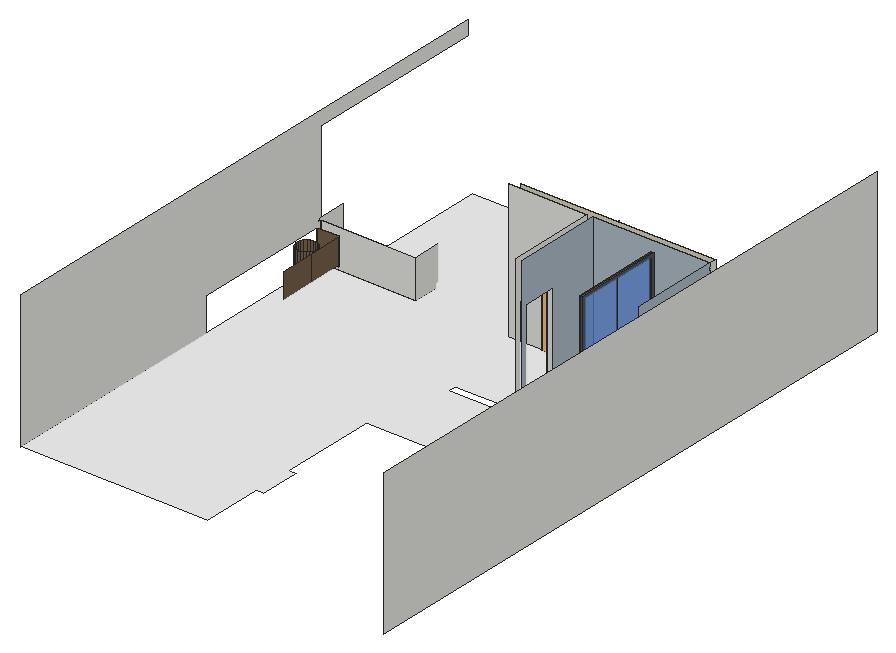
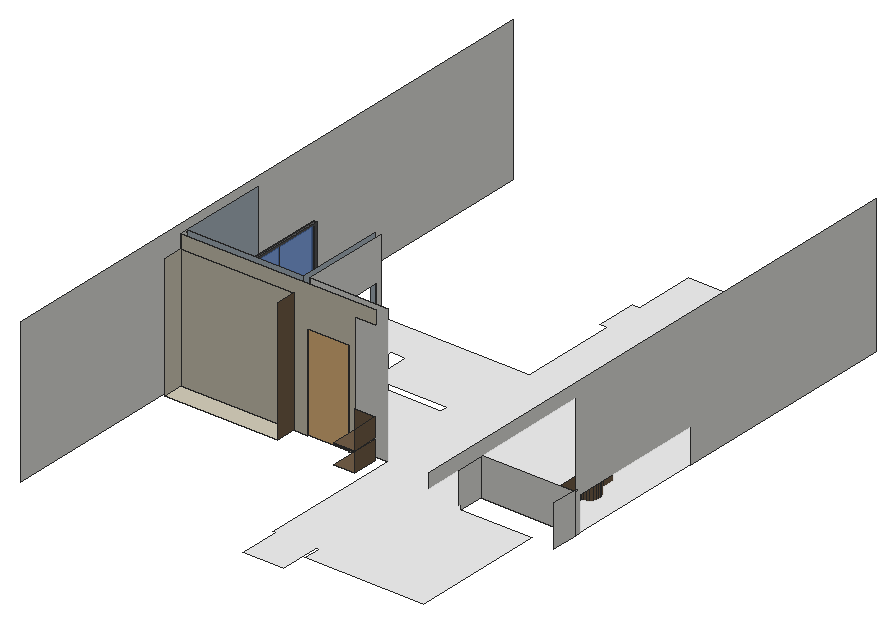
# SketchUp Ruby script. Lengths in inches.
U = 1.inch
M = Sketchup.active_model
def pt(a) = Geom::Point3d.new(a.map { |v| v * U })
def face(e, loops, mat)
  f = e.add_face(loops[0].map { |a| pt(a) })
  loops[1..].each { |l| e.add_face(l.map { |a| pt(a) }).erase! }
  f.material = f.back_material = mat if mat
  f
end
# faces: each face lists its corners as indices into pts; further lists are holes
def faces(e, pts, list, mat = nil) = list.each { |f| face(e, (f[0].is_a?(Array) ? f : [f]).map { |l| l.map { |i| pts[i] } }, mat) }
# xy, xz, yz: faces in a plane at the given z, y or x. An outline is a flat list of corners, or four numbers for a rectangle; further outlines are holes
def ring(l) = l.size == 4 ? [[l[0], l[1]], [l[2], l[1]], [l[2], l[3]], [l[0], l[3]]] : l.each_slice(2).to_a
def flat(e, list, mat, &to3) = list.each { |f| face(e, (f[0].is_a?(Array) ? f : [f]).map { |l| ring(l).map { |u, v| to3.(u, v) } }, mat) }
def xy(e, z, list, mat = nil) = flat(e, list, mat) { |x, y| [x, y, z] }
def xz(e, y, list, mat = nil) = flat(e, list, mat) { |x, z| [x, y, z] }
def yz(e, x, list, mat = nil) = flat(e, list, mat) { |y, z| [x, y, z] }
def lines(e, pts, list) = list.each { |a, b| e.add_line(pt(pts[a]), pt(pts[b])) }
# prism: a flat outline (further loops are holes) pulled along v
def prism(e, loops, v, mat = nil)
  f = face(e, loops, mat); d = Geom::Vector3d.new(v.map { |x| x * U })
  f.pushpull(f.normal.samedirection?(d) ? d.length : -d.length)
end
def box(e, o, s, mat = nil) = prism(e, [[o, [o[0] + s[0], o[1], o[2]], [o[0] + s[0], o[1] + s[1], o[2]], [o[0], o[1] + s[1], o[2]]]], [0, 0, s[2]], mat)
def at(x, y, z, deg = 0) = Geom::Transformation.translation(pt([x, y, z])) * Geom::Transformation.rotation(ORIGIN, Z_AXIS, deg.degrees)
def axes(o, x, y, z) = Geom::Transformation.new([*x, 0, *y, 0, *z, 0, *pt(o).to_a, 1])
def part(name) = M.definitions.add(name)
# library, detail: a bought-in or finely detailed component or shape, given as its bounding box
def library(name, o, s) = part(name).tap { |d| box(d.entities, o, s) }
def detail(e, o, s) = box(e.add_group.entities, o, s)
def put(e, d, t, mat = nil) = e.add_instance(d, t).tap { |i| i.material = mat if mat }
def group(e, t, mat = nil) = e.add_group.tap { |g| g.transformation = t; g.material = mat if mat }.entities
root = M.entities
M.materials.add("1689 AP 8482 GREY BUCK").color = [214, 207, 188]
M.materials.add("BRANCO").color = [255, 255, 255]
M.materials.add("CROMADO 2").color = [157, 160, 161]
M.materials.add("Tiles Grey 04 100cm").color = [119, 132, 150]
M.materials.add("Tiles K04 100cm").color = [171, 184, 194]
M.materials.add("Tiles Marble White 03 180cm").color = [241, 241, 241]
M.materials["Tiles Marble White 03 180cm"].alpha = 0.94
M.materials.add("Wood Pecan 33-21 150cm").color = [115, 94, 72]
M.materials.add("[Color M06]").color = [86, 86, 86]
M.materials.add("[Translucent Glass Blue]1").color = [100, 149, 237]
M.materials["[Translucent Glass Blue]1"].alpha = 0.5
c1 = part("Group\#31")
xy(c1.entities,0,[[0,0,2,78]],"[Color M06]")
xy(c1.entities,2,[[0,2,1,39],[1.5,2,2,39],[0,39,0.5,76],[1,39,2,76]],"[Color M06]")
xy(c1.entities,2,[[1,2,1.5,39],[0.5,39,1,76]],"[Translucent Glass Blue]1")
xy(c1.entities,108.71,[[0,2,1,39],[1.5,2,2,39],[0,39,0.5,76],[1,39,2,76]],"[Color M06]")
xy(c1.entities,108.71,[[1,2,1.5,39],[0.5,39,1,76]],"[Translucent Glass Blue]1")
xy(c1.entities,110.71,[[0,0,2,78]],"[Color M06]")
xz(c1.entities,0,[[0,0,2,110.71]],"[Color M06]")
xz(c1.entities,2,[[0,2,1,108.71],[1.5,2,2,108.71]],"[Color M06]")
xz(c1.entities,2,[[1,2,1.5,108.71]],"[Translucent Glass Blue]1")
xz(c1.entities,39,[[0.5,2,1,108.71],[1,2,1.5,108.71]],"[Translucent Glass Blue]1")
xz(c1.entities,76,[[0,2,0.5,108.71],[1,2,2,108.71]],"[Color M06]")
xz(c1.entities,76,[[0.5,2,1,108.71]],"[Translucent Glass Blue]1")
xz(c1.entities,78,[[0,0,2,110.71]],"[Color M06]")
yz(c1.entities,0,[[[0,0,78,110.71],[2,2,76,108.71]]],"[Color M06]")
yz(c1.entities,0.5,[[39,2,76,108.71]],"[Translucent Glass Blue]1")
yz(c1.entities,1,[[2,2,39,108.71],[39,2,76,108.71]],"[Translucent Glass Blue]1")
yz(c1.entities,1.5,[[2,2,39,108.71]],"[Translucent Glass Blue]1")
yz(c1.entities,2,[[[0,0,78,110.71],[2,2,76,108.71]]],"[Color M06]")
c2 = library("Group\#138",[0,0,0],[13.73,23.69,16.64])
c3 = library("Group\#175",[0,0,0],[4.31,6.23,4.8])
c4 = library("FamíliaGeometriaCombinação_251615-3D View\#2",[-254.64,-26270.28,78.31],[8392.13,24888.38,1235.26])
c5 = part("FamíliaGeometriaCombinação_97511-3D View\#1")
yz(c5.entities,7558.01,[[3406.91,1590.59,3286.24,1817.54,3119.79,2013.39,2915.27,2169.07,2682.16,2277.35,2274.61,2409.44,1863.61,2530.4,1775.08,2554.87,1761.54,2560.44,1749.79,2569.18,1740.55,2580.55,1734.39,2593.83,1726.84,2635.4,1730.23,2677.51,1744.34,2717.33,2578.96,2627.63,3407.55,2493.59,3753.07,1752.63]],"CROMADO 2")
yz(c5.entities,8187.93,[[3406.91,1590.59,3753.07,1752.63,3407.55,2493.59,2578.96,2627.63,1744.34,2717.33,1730.23,2677.51,1726.84,2635.4,1734.39,2593.83,1740.55,2580.55,1749.79,2569.18,1761.54,2560.44,1775.08,2554.87,1863.61,2530.4,2274.61,2409.44,2682.16,2277.35,2915.27,2169.07,3119.79,2013.39,3286.24,1817.54]],"CROMADO 2")
p = [[8187.93,3406.91,1590.59],[8187.93,3286.24,1817.54],[7558.01,3286.24,1817.54],[7558.01,3406.91,1590.59],[7558.01,3753.07,1752.63],[7566.125,3817.02,1782.57],
  [7589.86,3877.7,1810.97],[7628.02,3932.01,1836.39],[7678.45,3977.41,1857.65],[8067.3,3977.1875,1857.54],[8117.93,3932.01,1836.39],[8156.08,3877.7,1810.97],
  [8179.82,3817.02,1782.57],[8187.93,3753.07,1752.63],[7558.01,3407.55,2493.59],[7563.03,3475.375,2480.6],[8182.92,3475.375,2480.6],[8187.93,3407.55,2493.59],
  [7566.03,3817.04,1782.58],[8179.91,3817.04,1782.58],[7578.05,3541.64,2467.61],[8167.9,3541.64,2467.61],[7589.7,3877.77,1811],[8156.24,3877.77,1811],
  [7603.16,3604.85,2454.94],[8142.79,3604.85,2454.94],[7615.36,3629.11,2447.24],[8130.58,3629.11,2447.24],[7634.87,3671.32,2415.78],[8111.08,3671.32,2415.78],
  [7694.13,3851.52,2154.96],[8051.82,3851.52,2154.96],[7627.82,3932.15,1836.46],[8118.125,3932.15,1836.46],[7558.01,3119.79,2013.39],[8187.93,3119.79,2013.39],
  [8067.5,3977.41,1857.65],[8187.93,2915.27,2169.07],[7558.01,2915.27,2169.07],[8187.93,2682.16,2277.35],[7558.01,2682.16,2277.35],[8187.93,2274.61,2409.44],
  [7558.01,2274.61,2409.44],[8187.93,1863.61,2530.4],[7558.01,1863.61,2530.4],[7626.48,3651.58,2434.19],[8119.47,3651.58,2434.19],[7558.01,2578.96,2627.63],
  [8187.93,2578.96,2627.63],[8187.93,1775.08,2554.87],[7558.01,1775.08,2554.87],[8187.93,1761.54,2560.44],[7558.01,1761.54,2560.44],[7558.01,1749.79,2569.18],
  [8187.93,1749.79,2569.18],[8187.93,1740.55,2580.55],[7558.01,1740.55,2580.55],[7558.01,1734.39,2593.83],[8187.93,1734.39,2593.83],[7558.01,1726.84,2635.4],
  [8187.93,1726.84,2635.4],[7558.01,1744.34,2717.33],[8187.93,1744.34,2717.33],[8187.93,1730.23,2677.51],[7558.01,1730.23,2677.51]]
faces(c5.entities,p,[[0,1,2,3],[4,5,6,7,8,9,10,11,12,13,0,3],[14,15,4],[16,17,13],[18,4,15],[13,19,16],[20,18,15],[21,16,19],
  [22,18,20],[19,23,21],[20,24,22],[23,25,21],[22,24,26],[25,23,27],[22,26,28],[29,27,23],
  [28,30,22],[31,29,23],[22,30,32],[23,33,31],[34,2,1,35],[30,8,32],[33,36,31],[31,36,8,30],
  [35,37,38,34],[30,28,29,31],[37,39,40,38],[40,39,41,42],[43,44,42,41],[28,26,45],[29,46,27],[28,45,46,29],
  [27,46,45,26],[26,24,25,27],[25,24,47,48],[47,24,14],[48,17,25],[14,24,20],[25,17,21],[15,14,20],
  [21,17,16],[49,50,44,43],[49,51,52,50],[53,52,51,54],[54,55,56,53],[57,56,55,58],[59,57,58,60],[48,47,61,62],
  [60,63,64,59],[61,64,63,62]],"CROMADO 2")
c6 = part("FamíliaGeometriaCombinação_97510-3D View\#1")
p = [[7437.66,-650.83,702.01],[7870.94,-619.67,525.26],[7870.94,-757.69,1123.13],[8304.22,-650.83,702.01],[7870.94,2098.87,1152.89],[7540.91,2075.13,1287.51],
  [8200.97,2075.13,1287.51],[7258.1875,-726.07,1128.71],[8483.69,-726.07,1128.71],[7404.21,2017.82,1612.53],[8337.67,2017.82,1612.53],[7870.94,-832.47,1732.15],
  [7437.66,-801.31,1555.41],[8304.22,-801.31,1555.41],[7540.91,1960.52,1937.55],[8200.97,1960.52,1937.55],[7870.94,3537.43,1582.84],[7617.09,3511.98,1727.17],
  [8124.79,3511.98,1727.17],[7870.94,1936.78,2072.17],[7617.09,3461.08,2015.84],[7870.94,3435.63,2160.17],[8124.79,3461.08,2015.84]]
faces(c6.entities,p,[[0,1,2],[2,1,3],[4,1,0,5],[6,3,1,4],[2,7,0],[2,3,8],[9,5,0,7],[8,3,6,10],
  [2,11,12],[2,13,11],[2,12,7],[2,8,13],[7,12,14,9],[8,10,15,13],[5,16,4],[6,4,16],
  [17,5,9],[18,10,6],[17,16,5],[16,18,6],[19,14,12,11],[11,13,15,19],[18,16,17,20,21,22],[20,9,14],
  [22,15,10],[17,9,20],[22,10,18],[21,14,19],[15,21,19],[21,20,14],[22,21,15]],"CROMADO 2")
c7 = part("FamíliaGeometriaCombinação_240639-3D View")
xy(c7.entities,2221.34,[[-688.98,-689.37,688.98,688.98]],"CROMADO 2")
xy(c7.entities,2910.29,[[-688.98,-2854.33,-688.98,-1279.53,688.16,-1279.53,688.98,-2854.33]],"CROMADO 2")
xy(c7.entities,3107.14,[[-688.98,-2854.33,688.98,688.98]],"CROMADO 2")
xz(c7.entities,-2854.33,[[-688.98,2910.29,688.98,3107.14]],"CROMADO 2")
xz(c7.entities,688.98,[[-688.98,2221.34,688.98,3107.14]],"CROMADO 2")
yz(c7.entities,-688.98,[[-689.37,2221.34,-684.83,2368.07,-716.21,2511.48,-781.63,2642.9,-877.14,2754.39,-996.95,2839.21,-1133.84,2892.25,-1279.53,2910.29,-2854.33,2910.29,-2854.33,3107.14,688.98,3107.14,688.98,2221.34]],"CROMADO 2")
yz(c7.entities,688.98,[[-689.37,2221.34,688.98,2221.34,688.98,3107.14,-2854.33,3107.14,-2854.33,2910.29,-1279.53,2910.29,-1133.84,2892.25,-996.95,2839.21,-877.14,2754.39,-781.63,2642.9,-716.21,2511.48,-684.83,2368.07]],"CROMADO 2")
p = [[-688.98,-684.83,2368.07],[-688.98,-689.37,2221.34],[688.98,-689.37,2221.34],[688.98,-684.83,2368.07],[-688.98,-716.21,2511.48],[688.98,-716.21,2511.48],
  [-688.98,-781.63,2642.9],[688.98,-781.63,2642.9],[-688.98,-877.14,2754.39],[688.98,-877.14,2754.39],[-688.98,-996.95,2839.21],[688.98,-996.95,2839.21],
  [-688.98,-1133.84,2892.25],[688.98,-1133.84,2892.25],[688.16,-1279.53,2910.29],[-688.98,-1279.53,2910.29]]
faces(c7.entities,p,[[0,1,2,3],[4,0,3,5],[6,4,5,7],[8,6,7,9],[10,8,9,11],[12,10,11,13],[14,15,12,13]],"CROMADO 2")
c8 = library("Door+80x210",[17.88,40.74,0],[31.52,6.14,82.69])
xy(root,-4,[[303,291,351,369]],"Tiles Grey 04 100cm")
xy(root,0,[[252,375,351,392.7]],"1689 AP 8482 GREY BUCK")
xy(root,0,[[248,291,303,369]],"Tiles Grey 04 100cm")
xy(root,0,[[9,39.5,174,39.5,174,93,180,93,180,129,174,129,174,213,351,213,351,285,267,285,267,249,255,249,255,285,189.8125,285,189.8125,291,243,291,243,295,248,295,248,325,243,325,243,369,240,369,240,375,204,375,204,369,174,369,174,495,172,495,172,531,136,531,136,495,134,495,134,510,30,510,30,390,93,390,93,369,9,369]],"Tiles Marble White 03 180cm")
xy(root,2,[[180,376,198,398]],"Wood Pecan 33-21 150cm")
xy(root,7,[[28.39,333.67,28.6875,333.97]],"Wood Pecan 33-21 150cm")
xy(root,15.25,[[19.02,331.45,21.24,331.51,23.375,332.14,25.27,333.3,26.81,334.92,27.87,336.87,28.39,339.04,28.33,341.26,27.7,343.39,26.53,345.29,24.92,346.82,22.96,347.88,20.8,348.4,18.58,348.35,16.44,347.71,14.55,346.55,13.01,344.9375,11.95,342.98,11.43,340.82,11.49,338.59,12.125,336.46,13.29,334.5625,14.9,333.03,16.86,331.97]],"Wood Pecan 33-21 150cm")
xy(root,18.5,[[180,376,198,398]],"Wood Pecan 33-21 150cm")
xy(root,19.5,[[180,376,198,398]],"Wood Pecan 33-21 150cm")
xz(root,325,[[243,0,248,84]])
xz(root,333.67,[[28.39,7,28.6875,29]],"Wood Pecan 33-21 150cm")
xz(root,333.97,[[28.39,7,28.6875,29]],"Wood Pecan 33-21 150cm")
xz(root,364.7,[[9,6,28.6875,30]],"Wood Pecan 33-21 150cm")
xz(root,369,[[9,0,93,34],[174,0,204,0,204,84,240,84,240,0,243,0,243,120,174,120]])
xz(root,369,[[303,-4,351,-4,351,120,248,120,248,0,303,0]],"Tiles K04 100cm")
xz(root,375,[[198,0,198,108,180,108,180,120,351,120,351,108,252,108,252,0,240,0,240,84,204,84,204,0],[252,0,351,108]],"1689 AP 8482 GREY BUCK")
xz(root,376,[[180,2,198,18.5],[180,19.5,198,36]],"Wood Pecan 33-21 150cm")
yz(root,9,[[39.5,0,242.61,0,242.61,30,364.7,30,364.7,0,369,0,369,34,367,34,367,36,369,36,369,108,531,108,531,120,39.5,120],[369,0,393,0,393,36,367,36,367,34,369,34]])
yz(root,28.39,[[333.67,7,333.97,29]],"Wood Pecan 33-21 150cm")
yz(root,28.6875,[[303.65,7,333.67,29],[333.97,7,363.7,29]],"Wood Pecan 33-21 150cm")
yz(root,93,[[369,0,390,0,390,4,393,4,393,34,369,34]])
yz(root,180,[[376,2,398,18.5],[376,19.5,398,36]],"Wood Pecan 33-21 150cm")
yz(root,204,[[369,0,375,84]])
yz(root,240,[[369,0,375,84]])
yz(root,243,[[291,0,291,120,369,120,369,0,325,0,325,84,295,84,295,0]])
yz(root,248,[[291,0,295,0,295,84,325,84,325,0,369,0,369,120,291,120]],"Tiles K04 100cm")
yz(root,252,[[375,0,375,108,393,108,393,3,392.7,3,392.7,0]],"Wood Pecan 33-21 150cm")
yz(root,303,[[291,-4,369,0]],"Tiles Grey 04 100cm")
yz(root,351,[[369,0,375,120]])
yz(root,351,[[375,0,375,108,393,108,393,3,392.7,3,392.7,0]],"1689 AP 8482 GREY BUCK")
yz(root,351,[[291,-4,369,120]],"Tiles K04 100cm")
yz(root,360,[[0,-6,540,120]])
p = [[16.86,331.97,30],[19.02,331.45,30],[19.02,331.45,15.25],[16.86,331.97,15.25],[21.24,331.51,30],[21.24,331.51,15.25],
  [23.375,332.14,30],[23.375,332.14,15.25],[14.9,333.03,30],[14.9,333.03,15.25],[25.27,333.3,30],[25.27,333.3,15.25],
  [13.29,334.5625,30],[13.29,334.5625,15.25],[26.81,334.92,30],[26.81,334.92,15.25],[12.125,336.46,30],[12.125,336.46,15.25],
  [27.87,336.87,30],[27.87,336.87,15.25],[11.49,338.59,30],[11.49,338.59,15.25],[28.39,339.04,30],[28.39,339.04,15.25],
  [11.43,340.82,30],[11.43,340.82,15.25],[28.33,341.26,30],[28.33,341.26,15.25],[11.95,342.98,30],[11.95,342.98,15.25],
  [27.7,343.39,30],[27.7,343.39,15.25],[13.01,344.9375,30],[13.01,344.9375,15.25],[26.53,345.29,30],[26.53,345.29,15.25],
  [14.55,346.55,30],[14.55,346.55,15.25],[24.92,346.82,30],[24.92,346.82,15.25],[16.44,347.71,30],[16.44,347.71,15.25],
  [22.96,347.88,30],[22.96,347.88,15.25],[18.58,348.35,30],[18.58,348.35,15.25],[20.8,348.4,30],[20.8,348.4,15.25]]
faces(root,p,[[0,1,2,3],[1,4,5,2],[4,6,7,5],[8,0,3,9],[6,10,11,7],[12,8,9,13],[10,14,15,11],[16,12,13,17],
  [14,18,19,15],[20,16,17,21],[18,22,23,19],[24,20,21,25],[22,26,27,23],[28,24,25,29],[26,30,31,27],[32,28,29,33],
  [30,34,35,31],[36,32,33,37],[34,38,39,35],[40,36,37,41],[38,42,43,39],[44,40,41,45],[42,46,47,43],[46,44,45,47]],"Wood Pecan 33-21 150cm")
put(root,c1,at(299.29,291,0))
put(root,c2,at(266.64,348.75,0),"BRANCO")
put(root,c3,at(290.78,369,19.1,-90))
g1 = group(root,at(284.32,372.4375,0),"CROMADO 2")
put(g1,c4,axes([1.04,0,26.27],[0.001,0,0],[0,0,0.001],[0,-0.001,0]))
g2 = group(g1,at(8.25,0,21.82),"CROMADO 2")
put(g2,c5,axes([-7.2,0,4.45],[0.001,0,0],[0,0,0.001],[0,-0.001,0]))
put(g2,c6,axes([-7.2,0,4.45],[0.001,0,0],[0,0,0.001],[0,-0.001,0]))
g3 = group(g2,at(0.16,-0.49,7.36))
prism(g3,[[[0.87,-1.54,0.79],[0.51,-1.6,0.92],[0.15,-1.54,0.79],[0,-1.39,0.46],[0.15,-1.23,0.14],[0.51,-1.17,0],[0.87,-1.23,0.14],[1.02,-1.39,0.46]]],[0,1.17,0.55])
g4 = group(g2,at(0,0,4.2))
prism(g4,[[[0.29,-1.17,0],[0.21,-1.28,0],[0.15,-1.4,0],[0.14,-1.49,0],[0.14,-1.58,0],[0.17,-1.73,0],[0.09,-1.64,0],[0.04,-1.53,0],[0,-1.42,0],[0,0,0],[1.34,0,0],[1.34,-1.4,0],[1.31,-1.53,0],[1.25,-1.64,0],[1.17,-1.74,0],[1.2,-1.57,0],[1.2,-1.48,0],[1.18,-1.4,0],[1.13,-1.28,0],[1.04,-1.17,0],[0.93,-1.09,0],[0.8,-1.04,0],[0.67,-1.02,0],[0.53,-1.04,0],[0.41,-1.09,0]]],[0,0,0.97])
g5 = group(g2,at(0.38,-0.08,0))
p = [[0.05,-0.66,1.12],[0.12,-0.48,0.01],[0.21,-0.78,1.15],[0.18,-0.5,0],[0.24,-0.52,0],[0.34,-0.73,0.92],
  [0.07,-0.43,0.02],[0,-0.47,0.99],[0.01,-0.32,0.05],[0.03,-0.38,0.03],[0.31,-0.52,0],[0.375,-0.5,0],
  [0.43,-0.48,0.01],[0.5,-0.7,1.3],[0.48,-0.43,0.02],[0.55,-0.47,0.99],[0.52,-0.38,0.03],[0,-0.26,0.06],
  [0.54,-0.32,0.05],[0.55,-0.26,0.06],[0.03,-0.14,0.09],[0.01,-0.2,0.07],[0.05,-0.41,1.37],[0.5,-0.36,1.1875],
  [0.54,-0.2,0.07],[0.07,-0.09,0.1],[0.21,-0.22,1.04],[0.12,-0.04,0.11],[0.43,-0.04,0.11],[0.34,-0.27,1.26],
  [0.48,-0.09,0.1],[0.52,-0.14,0.09],[0.31,0,0.12],[0.375,-0.02,0.12],[0.18,-0.02,0.12],[0.24,0,0.12],
  [0.5,-0.99,2.54],[0.34,-0.94,1.86],[0.55,-0.91,2.86],[0.55,-0.69,1.92],[0,-0.91,2.86],[0.05,-0.69,2.61],
  [0,-0.69,1.92],[0.21,-0.4375,1.98],[0.23,-0.96,1.91],[0.09,-0.94,2.125],[0.02,-0.86,2.16],[0.53,-0.65,2.21],
  [0.46,-0.55,2.21],[0.32,-0.44,2.03],[0.21,-1.13,2.67],[0.4,-1.13,2.76],[0.15,-0.66,2.87],[0.34,-0.62,2.79],
  [0.05,-1.07,2.89],[0.5,-0.77,2.96],[0.48,-1.29,3.75],[0.52,-1.24,3.76],[0.54,-1.18,3.77],[0.01,-1.06,3.8],
  [0.03,-1,3.82],[0.07,-0.95,3.83],[0.18,-1.36,3.73],[0.12,-1.34,3.74],[0.24,-1.38,3.73],[0.31,-1.38,3.73],
  [0.375,-1.36,3.73],[0.43,-1.34,3.74],[0.24,-0.86,3.85],[0.31,-0.86,3.85],[0.375,-0.875,3.84],[0.43,-0.9,3.84],
  [0.07,-1.29,3.75],[0.03,-1.24,3.76],[0.01,-1.18,3.77],[0,-1.12,3.79],[0.55,-1.12,3.79],[0.54,-1.06,3.8],
  [0.18,-0.875,3.84],[0.12,-0.9,3.84],[0.52,-1,3.82],[0.48,-0.95,3.83]]
faces(g5,p,[[0,1,2],[3,2,1],[4,5,2],[4,2,3],[1,0,6],[0,7,8],[6,0,9],[8,9,0],
  [4,10,5],[5,11,12],[10,11,5],[5,12,13],[14,13,12],[15,13,16],[16,13,14],[8,7,17],
  [16,18,15],[18,19,15],[20,21,7],[7,22,20],[21,17,7],[23,15,24],[24,15,19],[20,22,25],
  [26,27,22],[25,22,27],[23,28,29],[28,23,30],[24,31,23],[30,23,31],[32,26,29],[32,29,33],
  [33,29,28],[26,34,27],[35,34,26],[32,35,26],[5,13,36,37],[5,37,2],[38,36,13,15,39],[40,41,22,7,42],
  [0,42,7],[26,22,41,43],[23,39,15],[26,43,29],[2,44,45],[37,44,2],[42,0,46],[0,2,45],
  [45,46,0],[39,23,47],[23,29,48],[48,47,23],[29,49,48],[43,49,29],[50,45,44],[37,51,50],
  [44,37,50],[37,36,51],[42,46,40],[39,47,38],[43,41,52],[43,52,53],[49,43,53],[53,48,49],
  [45,54,46],[54,45,50],[40,46,54],[38,47,55],[55,48,53],[48,55,47],[56,51,36],[36,57,56],
  [36,58,57],[36,38,58],[41,40,59],[41,59,60],[41,60,61],[61,52,41],[62,63,50],[64,50,65],
  [51,65,50],[50,64,62],[50,63,54],[66,65,51],[66,51,67],[67,51,56],[52,68,53],[69,53,68],
  [53,69,70],[53,71,55],[70,71,53],[54,63,72],[73,54,72],[40,74,75],[73,74,54],[40,54,74],
  [38,76,58],[40,75,59],[38,55,77],[38,77,76],[78,52,79],[79,52,61],[78,68,52],[80,77,55],
  [80,55,81],[55,71,81],[60,59,75,74,73,72,63,62,64,65,66,67,56,57,58,76,77,80,81,71,70,69,68,78,79,61]])
g6 = group(g1,at(0,0,23.42))
box(g6,[0.57,-2.22,2.38],[0.95,0.08,0.95])
put(g6,c7,axes([1.04,0,2.85],[0.001,0,0],[0,0,0.001],[0,-0.001,0]))
g7 = group(g6,at(0.56,-0.56,1.47))
xy(g7,0,[[0.49,-0.98,0.14,-0.83,0,-0.49,0.14,-0.14,0.49,0,0.83,-0.14,0.98,-0.49,0.83,-0.83]],"CROMADO 2")
xy(g7,0.39,[[[0.49,-0.98,0.83,-0.83,0.98,-0.49,0.83,-0.14,0.49,0,0.14,-0.14,0,-0.49,0.14,-0.83],[0.49,-0.89,0.14,-0.69,0.14,-0.28,0.49,-0.08,0.84,-0.28,0.84,-0.69]]],"CROMADO 2")
xy(g7,0.63,[[0.49,-0.89,0.84,-0.69,0.84,-0.28,0.49,-0.08,0.14,-0.28,0.14,-0.69]],"CROMADO 2")
yz(g7,0.14,[[-0.69,0.39,-0.28,0.63]],"CROMADO 2")
yz(g7,0.84,[[-0.69,0.39,-0.28,0.63]],"CROMADO 2")
p = [[0.49,-0.98,0.39],[0.14,-0.83,0.39],[0.14,-0.83,0],[0.49,-0.98,0],[0.83,-0.83,0.39],[0.83,-0.83,0],
  [0,-0.49,0],[0,-0.49,0.39],[0.98,-0.49,0.39],[0.98,-0.49,0],[0.14,-0.14,0.39],[0.14,-0.14,0],
  [0.83,-0.14,0],[0.83,-0.14,0.39],[0.49,0,0.39],[0.49,0,0],[0.49,-0.89,0.63],[0.14,-0.69,0.63],
  [0.14,-0.69,0.39],[0.49,-0.89,0.39],[0.84,-0.69,0.63],[0.84,-0.69,0.39],[0.14,-0.28,0.63],[0.49,-0.08,0.63],
  [0.49,-0.08,0.39],[0.14,-0.28,0.39],[0.84,-0.28,0.63],[0.84,-0.28,0.39]]
faces(g7,p,[[0,1,2,3],[4,0,3,5],[6,2,1,7],[8,4,5,9],[7,10,11,6],[9,12,13,8],[10,14,15,11],[14,13,12,15],
  [16,17,18,19],[20,16,19,21],[22,23,24,25],[23,26,27,24]],"CROMADO 2")
g8 = group(g6,at(0,0,1.8125))
box(g8,[0,-0.48,0],[2.09,0.48,2.09],"CROMADO 2")
g9 = group(g6,at(0.35,-0.48,2.11))
box(g9,[0,-1.66,0],[1.38,1.66,1.5],"CROMADO 2")
put(root,c8,axes([260.42,415.08,0],[-1.14198,0,0],[0,-1,0],[0,0,1.0158]))
